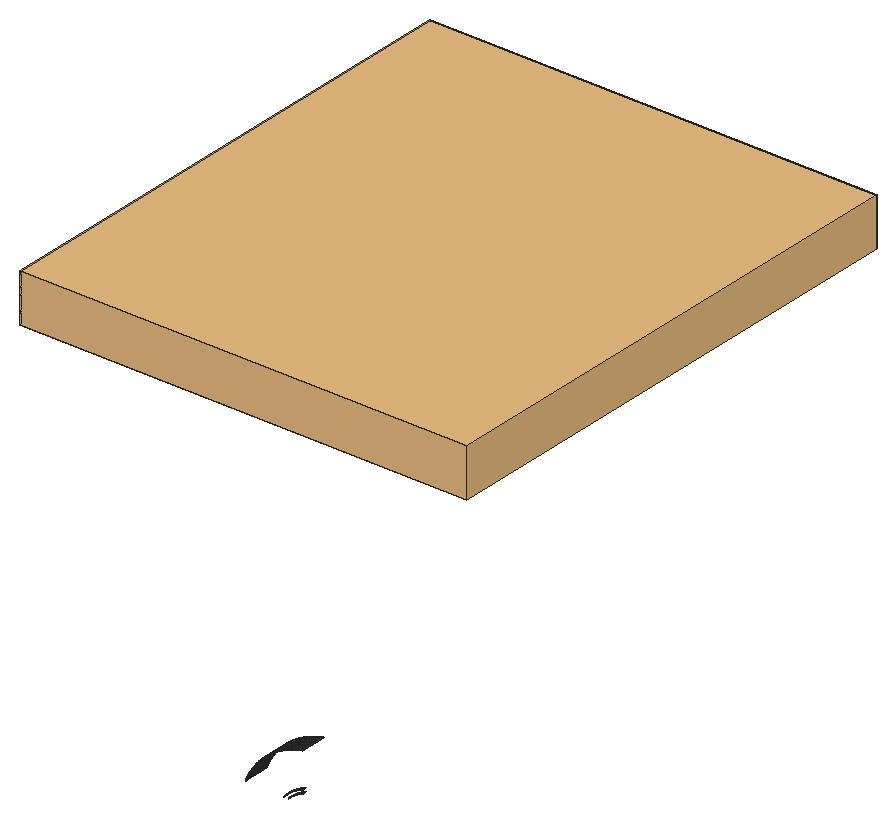
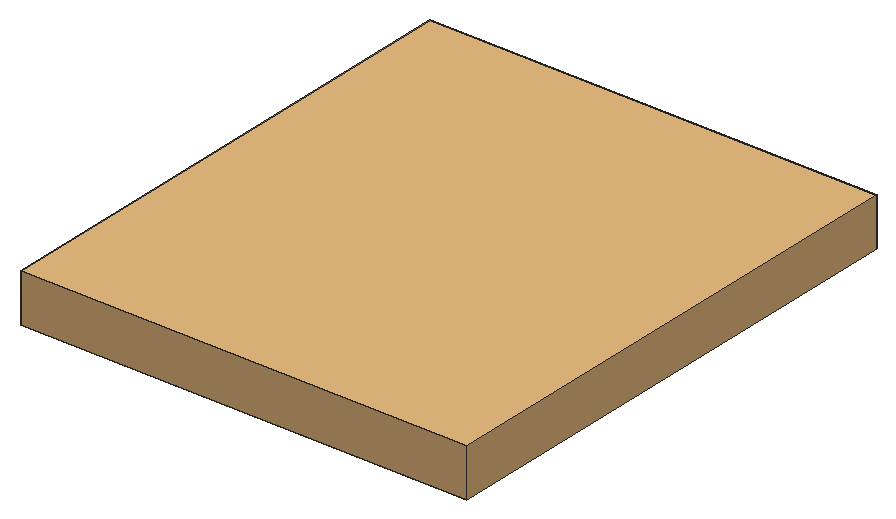
# SketchUp Ruby script. Lengths in inches.
U = 1.inch
M = Sketchup.active_model
def pt(a) = Geom::Point3d.new(a.map { |v| v * U })
def face(e, loops, mat)
  f = e.add_face(loops[0].map { |a| pt(a) })
  loops[1..].each { |l| e.add_face(l.map { |a| pt(a) }).erase! }
  f.material = f.back_material = mat if mat
  f
end
# faces: each face lists its corners as indices into pts; further lists are holes
def faces(e, pts, list, mat = nil) = list.each { |f| face(e, (f[0].is_a?(Array) ? f : [f]).map { |l| l.map { |i| pts[i] } }, mat) }
# xy, xz, yz: faces in a plane at the given z, y or x. An outline is a flat list of corners, or four numbers for a rectangle; further outlines are holes
def ring(l) = l.size == 4 ? [[l[0], l[1]], [l[2], l[1]], [l[2], l[3]], [l[0], l[3]]] : l.each_slice(2).to_a
def flat(e, list, mat, &to3) = list.each { |f| face(e, (f[0].is_a?(Array) ? f : [f]).map { |l| ring(l).map { |u, v| to3.(u, v) } }, mat) }
def xy(e, z, list, mat = nil) = flat(e, list, mat) { |x, y| [x, y, z] }
def xz(e, y, list, mat = nil) = flat(e, list, mat) { |x, z| [x, y, z] }
def yz(e, x, list, mat = nil) = flat(e, list, mat) { |y, z| [x, y, z] }
def lines(e, pts, list) = list.each { |a, b| e.add_line(pt(pts[a]), pt(pts[b])) }
# prism: a flat outline (further loops are holes) pulled along v
def prism(e, loops, v, mat = nil)
  f = face(e, loops, mat); d = Geom::Vector3d.new(v.map { |x| x * U })
  f.pushpull(f.normal.samedirection?(d) ? d.length : -d.length)
end
def box(e, o, s, mat = nil) = prism(e, [[o, [o[0] + s[0], o[1], o[2]], [o[0] + s[0], o[1] + s[1], o[2]], [o[0], o[1] + s[1], o[2]]]], [0, 0, s[2]], mat)
def at(x, y, z, deg = 0) = Geom::Transformation.translation(pt([x, y, z])) * Geom::Transformation.rotation(ORIGIN, Z_AXIS, deg.degrees)
def axes(o, x, y, z) = Geom::Transformation.new([*x, 0, *y, 0, *z, 0, *pt(o).to_a, 1])
def part(name) = M.definitions.add(name)
# library, detail: a bought-in or finely detailed component or shape, given as its bounding box
def library(name, o, s) = part(name).tap { |d| box(d.entities, o, s) }
def detail(e, o, s) = box(e.add_group.entities, o, s)
def put(e, d, t, mat = nil) = e.add_instance(d, t).tap { |i| i.material = mat if mat }
def group(e, t, mat = nil) = e.add_group.tap { |g| g.transformation = t; g.material = mat if mat }.entities
root = M.entities
M.materials.add("1432 AP 8245 TAR ROAD").color = [71, 72, 75]
M.materials.add("Outer Light").color = [251, 217, 152]
c1 = library("2",[-24,-36,-9.91],[204,234,21.91])
p = [[263.52,95.37,574.23],[263.41,95.37,574.11],[263.41,96.87,574.11],[263.52,96.87,574.23],[263.52,96.87,574.23],[263.41,96.87,574.11],
  [263.41,95.37,574.11],[263.52,95.37,574.23],[265.46,95.37,574.12],[265.56,95.37,574.23],[265.56,96.87,574.23],[265.46,96.87,574.12],
  [265.46,96.87,574.12],[265.56,96.87,574.23],[265.56,95.37,574.23],[265.46,95.37,574.12],[263.62,95.37,574.35],[263.62,96.87,574.35],
  [263.62,96.87,574.35],[263.62,95.37,574.35],[265.67,95.37,574.33],[265.67,96.87,574.33],[265.67,96.87,574.33],[265.67,95.37,574.33],
  [245.74,107.37,574.57],[245.63,107.37,574.31],[245.63,95.37,574.31],[245.74,95.37,574.57],[263.73,95.37,574.47],[263.73,96.87,574.47],
  [263.73,96.87,574.47],[263.73,95.37,574.47],[265.78,95.37,574.4375],[265.78,96.87,574.4375],[265.78,96.87,574.4375],[265.78,95.37,574.4375],
  [265.89,95.37,574.54],[265.89,96.87,574.54],[265.89,96.87,574.54],[265.89,95.37,574.54],[263.84,95.37,574.59],[263.84,96.87,574.59],
  [263.84,96.87,574.59],[263.84,95.37,574.59],[265.99,95.37,574.64],[265.99,96.87,574.64],[265.99,96.87,574.64],[265.99,95.37,574.64],
  [245.85,107.37,574.83],[245.85,95.37,574.83],[263.95,95.37,574.71],[263.95,96.87,574.71],[263.95,96.87,574.71],[263.95,95.37,574.71],
  [266.1,95.37,574.74],[266.1,96.87,574.74],[266.1,96.87,574.74],[266.1,95.37,574.74],[264.06,95.37,574.83],[264.06,96.87,574.83],
  [264.06,96.87,574.83],[264.06,95.37,574.83],[266.21,95.37,574.85],[266.21,96.87,574.85],[266.21,96.87,574.85],[266.21,95.37,574.85],
  [245.96,107.37,575.09],[245.96,95.37,575.09],[264.17,95.37,574.94],[264.17,96.87,574.94],[264.17,96.87,574.94],[264.17,95.37,574.94],
  [266.32,95.37,574.95],[266.32,96.87,574.95],[266.32,96.87,574.95],[266.32,95.37,574.95],[264.28,95.37,575.06],[264.28,96.87,575.06],
  [264.28,96.87,575.06],[264.28,95.37,575.06],[266.44,95.37,575.04],[266.44,96.87,575.04],[266.44,96.87,575.04],[266.44,95.37,575.04],
  [266.55,95.37,575.14],[266.55,96.87,575.14],[266.55,96.87,575.14],[266.55,95.37,575.14],[246.07,107.37,575.35],[246.07,95.37,575.35],
  [264.39,95.37,575.17],[264.39,96.87,575.17],[264.39,96.87,575.17],[264.39,95.37,575.17],[266.66,95.37,575.24],[266.66,96.87,575.24],
  [266.66,96.87,575.24],[266.66,95.37,575.24],[264.5,95.37,575.29],[264.5,96.87,575.29],[264.5,96.87,575.29],[264.5,95.37,575.29],
  [266.77,95.37,575.34],[266.77,96.87,575.34],[266.77,96.87,575.34],[266.77,95.37,575.34],[246.1875,107.37,575.61],[246.1875,95.37,575.61],
  [264.62,95.37,575.4],[264.62,96.87,575.4],[264.62,96.87,575.4],[264.62,95.37,575.4],[266.89,95.37,575.43],[266.89,96.87,575.43],
  [266.89,96.87,575.43],[266.89,95.37,575.43],[264.73,95.37,575.51],[264.73,96.87,575.51],[264.73,96.87,575.51],[264.73,95.37,575.51],
  [267,95.37,575.53],[267,96.87,575.53],[267,96.87,575.53],[267,95.37,575.53],[264.85,95.37,575.625],[264.85,96.87,575.625],
  [264.85,96.87,575.625],[264.85,95.37,575.625],[267.12,95.37,575.62],[267.12,96.87,575.62],[267.12,96.87,575.62],[267.12,95.37,575.62],
  [246.31,107.37,575.86],[246.31,95.37,575.86],[264.97,95.37,575.74],[264.97,96.87,575.74],[264.97,96.87,575.74],[264.97,95.37,575.74],
  [267.24,95.37,575.71],[267.24,96.87,575.71],[267.24,96.87,575.71],[267.24,95.37,575.71],[265.08,95.37,575.85],[265.08,96.87,575.85],
  [265.08,96.87,575.85],[265.08,95.37,575.85],[267.35,95.37,575.8],[267.35,96.87,575.8],[267.35,96.87,575.8],[267.35,95.37,575.8],
  [265.2,95.37,575.95],[265.2,96.87,575.95],[265.2,96.87,575.95],[265.2,95.37,575.95],[267.47,95.37,575.9],[267.47,96.87,575.9],
  [267.47,96.87,575.9],[267.47,95.37,575.9],[246.43,107.37,576.12],[246.43,95.37,576.12],[267.59,95.37,575.99],[267.59,96.87,575.99],
  [267.59,96.87,575.99],[267.59,95.37,575.99],[265.32,95.37,576.0625],[265.32,96.87,576.0625],[265.32,96.87,576.0625],[265.32,95.37,576.0625],
  [267.71,95.37,576.08],[267.71,96.87,576.08],[267.71,96.87,576.08],[267.71,95.37,576.08],[246.55,107.37,576.375],[246.55,95.37,576.375],
  [265.44,95.37,576.17],[265.44,96.87,576.17],[265.44,96.87,576.17],[265.44,95.37,576.17],[267.83,95.37,576.16],[267.83,96.87,576.16],
  [267.83,96.87,576.16],[267.83,95.37,576.16],[265.5625,95.37,576.28],[265.5625,96.87,576.28],[265.5625,96.87,576.28],[265.5625,95.37,576.28],
  [267.95,95.37,576.25],[267.95,96.87,576.25],[267.95,96.87,576.25],[267.95,95.37,576.25],[265.6875,95.37,576.38],[265.6875,96.87,576.38],
  [265.6875,96.87,576.38],[265.6875,95.37,576.38],[268.07,95.37,576.34],[268.07,96.87,576.34],[268.07,96.87,576.34],[268.07,95.37,576.34],
  [268.2,95.37,576.42],[268.2,96.87,576.42],[268.2,96.87,576.42],[268.2,95.37,576.42],[246.67,107.37,576.63],[246.67,95.37,576.63],
  [265.81,95.37,576.48],[265.81,96.87,576.48],[265.81,96.87,576.48],[265.81,95.37,576.48],[268.32,95.37,576.51],[268.32,96.87,576.51],
  [268.32,96.87,576.51],[268.32,95.37,576.51],[265.93,95.37,576.59],[265.93,96.87,576.59],[265.93,96.87,576.59],[265.93,95.37,576.59],
  [268.44,95.37,576.59],[268.44,96.87,576.59],[268.44,96.87,576.59],[268.44,95.37,576.59],[246.8,107.37,576.88],[246.8,95.37,576.88],
  [266.06,95.37,576.69],[266.06,96.87,576.69],[266.06,96.87,576.69],[266.06,95.37,576.69],[268.57,95.37,576.67],[268.57,96.87,576.67],
  [268.57,96.87,576.67],[268.57,95.37,576.67],[266.18,95.37,576.79],[266.18,96.87,576.79],[266.18,96.87,576.79],[266.18,95.37,576.79],
  [268.69,95.37,576.75],[268.69,96.87,576.75],[268.69,96.87,576.75],[268.69,95.37,576.75],[266.31,95.37,576.89],[266.31,96.87,576.89],
  [266.31,96.87,576.89],[266.31,95.37,576.89],[268.82,95.37,576.83],[268.82,96.87,576.83],[268.82,96.87,576.83],[268.82,95.37,576.83],
  [268.95,95.37,576.91],[268.95,96.87,576.91],[268.95,96.87,576.91],[268.95,95.37,576.91],[246.92,107.37,577.14],[246.92,95.37,577.14],
  [266.44,95.37,576.99],[266.44,96.87,576.99],[266.44,96.87,576.99],[266.44,95.37,576.99],[269.07,95.37,576.99],[269.07,96.87,576.99],
  [269.07,96.87,576.99],[269.07,95.37,576.99],[266.5625,95.37,577.09],[266.5625,96.87,577.09],[266.5625,96.87,577.09],[266.5625,95.37,577.09],
  [269.2,95.37,577.07],[269.2,96.87,577.07],[269.2,96.87,577.07],[269.2,95.37,577.07],[247.05,107.37,577.39],[247.05,95.37,577.39],
  [266.69,95.37,577.1875],[266.69,96.87,577.1875],[266.69,96.87,577.1875],[266.69,95.37,577.1875],[269.33,95.37,577.15],[269.33,96.87,577.15],
  [269.33,96.87,577.15],[269.33,95.37,577.15],[269.46,95.37,577.22],[269.46,96.87,577.22],[269.46,96.87,577.22],[269.46,95.37,577.22],
  [266.82,95.37,577.28],[266.82,96.87,577.28],[266.82,96.87,577.28],[266.82,95.37,577.28],[269.59,95.37,577.3],[269.59,96.87,577.3],
  [269.59,96.87,577.3],[269.59,95.37,577.3],[266.95,95.37,577.375],[266.95,96.87,577.375],[266.95,96.87,577.375],[266.95,95.37,577.375],
  [269.72,95.37,577.37],[269.72,96.87,577.37],[269.72,96.87,577.37],[269.72,95.37,577.37],[247.18,107.37,577.64],[247.18,95.37,577.64],
  [267.08,95.37,577.47],[267.08,96.87,577.47],[267.08,96.87,577.47],[267.08,95.37,577.47],[269.85,95.37,577.44],[269.85,96.87,577.44],
  [269.85,96.87,577.44],[269.85,95.37,577.44],[269.98,95.37,577.51],[269.98,96.87,577.51],[269.98,96.87,577.51],[269.98,95.37,577.51],
  [267.21,95.37,577.5625],[267.21,96.87,577.5625],[267.21,96.87,577.5625],[267.21,95.37,577.5625],[270.11,95.37,577.58],[270.11,96.87,577.58],
  [270.11,96.87,577.58],[270.11,95.37,577.58],[247.32,107.37,577.89],[247.32,95.37,577.89],[267.34,95.37,577.66],[267.34,96.87,577.66],
  [267.34,96.87,577.66],[267.34,95.37,577.66],[270.24,95.37,577.65],[270.24,96.87,577.65],[270.24,96.87,577.65],[270.24,95.37,577.65],
  [267.48,95.37,577.75],[267.48,96.87,577.75],[267.48,96.87,577.75],[267.48,95.37,577.75],[267.61,95.37,577.84],[267.61,96.87,577.84],
  [267.61,96.87,577.84],[267.61,95.37,577.84],[270.375,95.37,577.72],[270.375,96.87,577.72],[270.375,96.87,577.72],[270.375,95.37,577.72],
  [270.51,95.37,577.79],[270.51,96.87,577.79],[270.51,96.87,577.79],[270.51,95.37,577.79],[267.75,95.37,577.93],[267.75,96.87,577.93],
  [267.75,96.87,577.93],[267.75,95.37,577.93],[270.64,95.37,577.85],[270.64,96.87,577.85],[270.64,96.87,577.85],[270.64,95.37,577.85],
  [247.45,107.37,578.14],[247.45,95.37,578.14],[267.88,95.37,578.01],[267.88,96.87,578.01],[267.88,96.87,578.01],[267.88,95.37,578.01],
  [270.78,95.37,577.92],[270.78,96.87,577.92],[270.78,96.87,577.92],[270.78,95.37,577.92],[270.91,95.37,577.98],[270.91,96.87,577.98],
  [270.91,96.87,577.98],[270.91,95.37,577.98],[268.02,95.37,578.1],[268.02,96.87,578.1],[268.02,96.87,578.1],[268.02,95.37,578.1],
  [271.05,95.37,578.05],[271.05,96.87,578.05],[271.05,96.87,578.05],[271.05,95.37,578.05],[271.18,95.37,578.11],[271.18,96.87,578.11],
  [271.18,96.87,578.11],[271.18,95.37,578.11],[247.59,107.37,578.38],[247.59,95.37,578.38],[268.15,95.37,578.1875],[268.15,96.87,578.1875],
  [268.15,96.87,578.1875],[268.15,95.37,578.1875],[271.32,95.37,578.17],[271.32,96.87,578.17],[271.32,96.87,578.17],[271.32,95.37,578.17],
  [268.29,95.37,578.27],[268.29,96.87,578.27],[268.29,96.87,578.27],[268.29,95.37,578.27],[271.45,95.37,578.23],[271.45,96.87,578.23],
  [271.45,96.87,578.23],[271.45,95.37,578.23],[271.59,95.37,578.29],[271.59,96.87,578.29],[271.59,96.87,578.29],[271.59,95.37,578.29],
  [268.43,95.37,578.35],[268.43,96.87,578.35],[268.43,96.87,578.35],[268.43,95.37,578.35],[271.73,95.37,578.35],[271.73,96.87,578.35],
  [271.73,96.87,578.35],[271.73,95.37,578.35],[271.87,95.37,578.4],[271.87,96.87,578.4],[271.87,96.87,578.4],[271.87,95.37,578.4],
  [247.73,107.37,578.63],[247.73,95.37,578.63],[268.56,95.37,578.4375],[268.56,96.87,578.4375],[268.56,96.87,578.4375],[268.56,95.37,578.4375],
  [268.7,95.37,578.52],[268.7,96.87,578.52],[268.7,96.87,578.52],[268.7,95.37,578.52],[272.01,95.37,578.46],[272.01,96.87,578.46],
  [272.01,96.87,578.46],[272.01,95.37,578.46],[268.84,95.37,578.6],[268.84,96.87,578.6],[268.84,96.87,578.6],[268.84,95.37,578.6],
  [247.87,107.37,578.875],[247.87,95.37,578.875],[268.98,95.37,578.68],[268.98,96.87,578.68],[268.98,96.87,578.68],[268.98,95.37,578.68],
  [269.125,95.37,578.76],[269.125,96.87,578.76],[269.125,96.87,578.76],[269.125,95.37,578.76],[269.27,95.37,578.83],[269.27,96.87,578.83],
  [269.27,96.87,578.83],[269.27,95.37,578.83],[269.41,95.37,578.91],[269.41,96.87,578.91],[269.41,96.87,578.91],[269.41,95.37,578.91],
  [248.01,107.37,579.12],[248.01,95.37,579.12],[269.55,95.37,578.98],[269.55,96.87,578.98],[269.55,96.87,578.98],[269.55,95.37,578.98],
  [269.69,95.37,579.06],[269.69,96.87,579.06],[269.69,96.87,579.06],[269.69,95.37,579.06],[248.16,107.37,579.36],[248.16,95.37,579.36],
  [269.84,95.37,579.13],[269.84,96.87,579.13],[269.84,96.87,579.13],[269.84,95.37,579.13],[269.98,95.37,579.2],[269.98,96.87,579.2],
  [269.98,96.87,579.2],[269.98,95.37,579.2],[270.125,95.37,579.27],[270.125,96.87,579.27],[270.125,96.87,579.27],[270.125,95.37,579.27],
  [270.27,95.37,579.34],[270.27,96.87,579.34],[270.27,96.87,579.34],[270.27,95.37,579.34],[270.42,95.37,579.41],[270.42,96.87,579.41],
  [270.42,96.87,579.41],[270.42,95.37,579.41],[248.3,107.37,579.6],[248.3,95.37,579.6],[270.5625,95.37,579.48],[270.5625,96.87,579.48],
  [270.5625,96.87,579.48],[270.5625,95.37,579.48],[270.71,95.37,579.54],[270.71,96.87,579.54],[270.71,96.87,579.54],[270.71,95.37,579.54],
  [270.86,95.37,579.61],[270.86,96.87,579.61],[270.86,96.87,579.61],[270.86,95.37,579.61],[248.45,107.37,579.84],[248.45,95.37,579.84],
  [271.01,95.37,579.67],[271.01,96.87,579.67],[271.01,96.87,579.67],[271.01,95.37,579.67],[271.15,95.37,579.73],[271.15,96.87,579.73],
  [271.15,96.87,579.73],[271.15,95.37,579.73],[271.3,95.37,579.79],[271.3,96.87,579.79],[271.3,96.87,579.79],[271.3,95.37,579.79],
  [248.6,107.37,580.08],[248.6,95.37,580.08],[271.45,95.37,579.85],[271.45,96.87,579.85],[271.45,96.87,579.85],[271.45,95.37,579.85],
  [271.6,95.37,579.91],[271.6,96.87,579.91],[271.6,96.87,579.91],[271.6,95.37,579.91],[271.75,95.37,579.97],[271.75,96.87,579.97],
  [271.75,96.87,579.97],[271.75,95.37,579.97],[271.9,95.37,580.02],[271.9,96.87,580.02],[271.9,96.87,580.02],[271.9,95.37,580.02],
  [272.06,95.37,580.08],[272.06,96.87,580.08],[248.76,107.37,580.32],[248.76,95.37,580.32],[248.91,107.37,580.56],[248.91,95.37,580.56],
  [249.07,107.37,580.79],[249.07,95.37,580.79],[249.23,107.37,581.03],[249.23,95.37,581.03],[249.38,107.37,581.26],[249.38,95.37,581.26],
  [249.55,107.37,581.49],[249.55,95.37,581.49],[249.71,107.37,581.72],[249.71,95.37,581.72],[249.875,107.37,581.95],[249.875,95.37,581.95],
  [250.04,107.37,582.18],[250.04,95.37,582.18],[250.21,107.37,582.41],[250.21,95.37,582.41],[250.38,107.37,582.63],[250.38,95.37,582.63],
  [250.55,107.37,582.86],[250.55,95.37,582.86],[250.73,107.37,583.08],[250.73,95.37,583.08],[250.9,107.37,583.3],[250.9,95.37,583.3],
  [251.08,107.37,583.52],[251.08,95.37,583.52],[251.26,107.37,583.74],[251.26,95.37,583.74],[251.44,107.37,583.96],[251.44,95.37,583.96],
  [251.625,107.37,584.17],[251.625,95.37,584.17],[251.81,107.37,584.39],[251.81,95.37,584.39],[252,107.37,584.6],[252,95.37,584.6],
  [252.18,107.37,584.8125],[252.18,95.37,584.8125],[252.375,107.37,585.02],[252.375,95.37,585.02],[252.5625,107.37,585.23],[252.5625,95.37,585.23],
  [252.76,107.37,585.4375],[252.76,95.37,585.4375],[252.95,107.37,585.64],[252.95,95.37,585.64],[253.15,107.37,585.84],[253.15,95.37,585.84],
  [253.35,107.37,586.05],[253.35,95.37,586.05],[253.54,107.37,586.25],[253.54,95.37,586.25],[253.74,107.37,586.45],[253.74,95.37,586.45],
  [253.95,107.37,586.64],[253.95,95.37,586.64],[254.15,107.37,586.84],[254.15,95.37,586.84],[254.36,107.37,587.03],[254.36,95.37,587.03],
  [254.5625,107.37,587.23],[254.5625,95.37,587.23],[254.77,107.37,587.42],[254.77,95.37,587.42],[254.98,107.37,587.61],[254.98,95.37,587.61],
  [255.19,107.37,587.8],[255.19,95.37,587.8],[255.41,107.37,587.98],[255.41,95.37,587.98],[255.62,107.37,588.17],[255.62,95.37,588.17],
  [255.84,107.37,588.35],[255.84,95.37,588.35],[256.05,107.37,588.53],[256.05,95.37,588.53],[256.27,107.37,588.71],[256.27,95.37,588.71],
  [256.49,107.37,588.89],[256.49,95.37,588.89],[256.71,107.37,589.0625],[256.71,95.37,589.0625],[256.94,107.37,589.24],[256.94,95.37,589.24],
  [257.16,107.37,589.41],[257.16,95.37,589.41],[257.38,107.37,589.58],[257.38,95.37,589.58],[257.61,107.37,589.75],[257.61,95.37,589.75],
  [257.84,107.37,589.92],[257.84,95.37,589.92],[258.07,107.37,590.08],[258.07,95.37,590.08],[258.3,107.37,590.25],[258.3,95.37,590.25],
  [258.53,107.37,590.41],[258.53,95.37,590.41],[258.76,107.37,590.57],[258.76,95.37,590.57],[259,107.37,590.72],[259,95.37,590.72],
  [259.24,107.37,590.88],[259.24,95.37,590.88],[259.47,107.37,591.04],[259.47,95.37,591.04],[259.71,107.37,591.1875],[259.71,95.37,591.1875],
  [259.95,107.37,591.34],[259.95,95.37,591.34],[260.19,107.37,591.49],[260.19,95.37,591.49],[260.43,107.37,591.63],[260.43,95.37,591.63],
  [260.67,107.37,591.78],[260.67,95.37,591.78],[260.92,107.37,591.92],[260.92,95.37,591.92],[261.16,107.37,592.0625],[261.16,95.37,592.0625],
  [261.41,107.37,592.2],[261.41,95.37,592.2],[261.66,107.37,592.34],[261.66,95.37,592.34],[261.91,107.37,592.47],[261.91,95.37,592.47],
  [262.15,107.37,592.61],[262.15,95.37,592.61],[262.4,107.37,592.74],[262.4,95.37,592.74],[262.66,107.37,592.87],[262.66,95.37,592.87],
  [262.91,107.37,593],[262.91,95.37,593],[263.16,107.37,593.12],[263.16,95.37,593.12],[263.42,107.37,593.24],[263.42,95.37,593.24],
  [263.67,107.37,593.37],[263.67,95.37,593.37],[263.93,107.37,593.49],[263.93,95.37,593.49],[264.19,107.37,593.6],[264.19,95.37,593.6],
  [264.44,107.37,593.72],[264.44,95.37,593.72],[264.7,107.37,593.83],[264.7,95.37,593.83],[264.96,107.37,593.94],[264.96,95.37,593.94],
  [265.22,107.37,594.05],[265.22,95.37,594.05],[265.49,107.37,594.16],[265.49,95.37,594.16],[265.75,107.37,594.26],[265.75,95.37,594.26],
  [266.01,107.37,594.37],[266.01,95.37,594.37],[266.27,107.37,594.47],[266.27,95.37,594.47],[266.54,107.37,594.57],[266.54,95.37,594.57],
  [266.81,107.37,594.66],[266.81,95.37,594.66],[267.07,107.37,594.76],[267.07,95.37,594.76],[267.34,107.37,594.85],[267.34,95.37,594.85],
  [267.61,107.37,594.94],[267.61,95.37,594.94],[267.875,107.37,595.03],[267.875,95.37,595.03],[268.14,107.37,595.12],[268.14,95.37,595.12],
  [268.41,107.37,595.2],[268.41,95.37,595.2],[268.69,107.37,595.28],[268.69,95.37,595.28],[268.96,107.37,595.36],[268.96,95.37,595.36],
  [269.23,107.37,595.44],[269.23,95.37,595.44],[269.5,107.37,595.52],[269.5,95.37,595.52],[269.77,107.37,595.59],[269.77,95.37,595.59],
  [270.05,107.37,595.66],[270.05,95.37,595.66],[270.32,107.37,595.73],[270.32,95.37,595.73],[270.6,107.37,595.8],[270.6,95.37,595.8],
  [270.87,107.37,595.86],[270.87,95.37,595.86],[271.15,107.37,595.93],[271.15,95.37,595.93],[271.42,107.37,595.99],[271.42,95.37,595.99],
  [271.7,107.37,596.04],[271.7,95.37,596.04],[271.98,107.37,596.1],[271.98,95.37,596.1]]
faces(root,p,[[0,1,2,3],[8,9,10,11],[16,0,3,17],[9,20,21,10],[24,25,26,27],[28,16,17,29],[20,32,33,21],[32,36,37,33],
  [40,28,29,41],[36,44,45,37],[48,24,27,49],[50,40,41,51],[44,54,55,45],[58,50,51,59],[54,62,63,55],[66,48,49,67],
  [68,58,59,69],[62,72,73,63],[76,68,69,77],[72,80,81,73],[80,84,85,81],[88,66,67,89],[90,76,77,91],[84,94,95,85],
  [98,90,91,99],[94,102,103,95],[106,88,89,107],[108,98,99,109],[102,112,113,103],[116,108,109,117],[112,120,121,113],[124,116,117,125],
  [120,128,129,121],[132,106,107,133],[134,124,125,135],[128,138,139,129],[142,134,135,143],[138,146,147,139],[150,142,143,151],[146,154,155,147],
  [158,132,133,159],[154,160,161,155],[164,150,151,165],[160,168,169,161],[172,158,159,173],[174,164,165,175],[168,178,179,169],[182,174,175,183],
  [178,186,187,179],[190,182,183,191],[186,194,195,187],[194,198,199,195],[202,172,173,203],[204,190,191,205],[198,208,209,199],[212,204,205,213],
  [208,216,217,209],[220,202,203,221],[222,212,213,223],[216,226,227,217],[230,222,223,231],[226,234,235,227],[238,230,231,239],[234,242,243,235],
  [242,246,247,243],[250,220,221,251],[252,238,239,253],[246,256,257,247],[260,252,253,261],[256,264,265,257],[268,250,251,269],[270,260,261,271],
  [264,274,275,265],[274,278,279,275],[282,270,271,283],[278,286,287,279],[290,282,283,291],[286,294,295,287],[298,268,269,299],[300,290,291,301],
  [294,304,305,295],[304,308,309,305],[312,300,301,313],[308,316,317,309],[320,298,299,321],[322,312,313,323],[316,326,327,317],[330,322,323,331],
  [334,330,331,335],[326,338,339,327],[338,342,343,339],[346,334,335,347],[342,350,351,343],[354,320,321,355],[356,346,347,357],[350,360,361,351],
  [360,364,365,361],[368,356,357,369],[364,372,373,365],[372,376,377,373],[380,354,355,381],[382,368,369,383],[376,386,387,377],[390,382,383,391],
  [386,394,395,387],[394,398,399,395],[402,390,391,403],[398,406,407,399],[406,410,411,407],[414,380,381,415],[416,402,403,417],[420,416,417,421],
  [410,424,425,411],[428,420,421,429],[432,414,415,433],[434,428,429,435],[438,434,435,439],[442,438,439,443],[446,442,443,447],[450,432,433,451],
  [452,446,447,453],[456,452,453,457],[460,450,451,461],[462,456,457,463],[466,462,463,467],[470,466,467,471],[474,470,471,475],[478,474,475,479],
  [482,460,461,483],[484,478,479,485],[488,484,485,489],[492,488,489,493],[496,482,483,497],[498,492,493,499],[502,498,499,503],[506,502,503,507],
  [510,496,497,511],[512,506,507,513],[516,512,513,517],[520,516,517,521],[524,520,521,525],[528,524,525,529],[530,510,511,531],[532,530,531,533],
  [534,532,533,535],[536,534,535,537],[538,536,537,539],[540,538,539,541],[542,540,541,543],[544,542,543,545],[546,544,545,547],[548,546,547,549],
  [550,548,549,551],[552,550,551,553],[554,552,553,555],[556,554,555,557],[558,556,557,559],[560,558,559,561],[562,560,561,563],[564,562,563,565],
  [566,564,565,567],[568,566,567,569],[570,568,569,571],[572,570,571,573],[574,572,573,575],[576,574,575,577],[578,576,577,579],[580,578,579,581],
  [582,580,581,583],[584,582,583,585],[586,584,585,587],[588,586,587,589],[590,588,589,591],[592,590,591,593],[594,592,593,595],[596,594,595,597],
  [598,596,597,599],[600,598,599,601],[602,600,601,603],[604,602,603,605],[606,604,605,607],[608,606,607,609],[610,608,609,611],[612,610,611,613],
  [614,612,613,615],[616,614,615,617],[618,616,617,619],[620,618,619,621],[622,620,621,623],[624,622,623,625],[626,624,625,627],[628,626,627,629],
  [630,628,629,631],[632,630,631,633],[634,632,633,635],[636,634,635,637],[638,636,637,639],[640,638,639,641],[642,640,641,643],[644,642,643,645],
  [646,644,645,647],[648,646,647,649],[650,648,649,651],[652,650,651,653],[654,652,653,655],[656,654,655,657],[658,656,657,659],[660,658,659,661],
  [662,660,661,663],[664,662,663,665],[666,664,665,667],[668,666,667,669],[670,668,669,671],[672,670,671,673],[674,672,673,675],[676,674,675,677],
  [678,676,677,679],[680,678,679,681],[682,680,681,683],[684,682,683,685],[686,684,685,687],[688,686,687,689],[690,688,689,691],[692,690,691,693],
  [694,692,693,695],[696,694,695,697],[698,696,697,699],[700,698,699,701],[702,700,701,703],[704,702,703,705],[706,704,705,707],[708,706,707,709],
  [710,708,709,711],[712,710,711,713],[714,712,713,715],[716,714,715,717],[718,716,717,719],[720,718,719,721],[722,720,721,723],[724,722,723,725],
  [726,724,725,727],[728,726,727,729],[730,728,729,731],[732,730,731,733],[734,732,733,735]],"1432 AP 8245 TAR ROAD")
faces(root,p,[[4,5,6,7],[12,13,14,15],[18,4,7,19],[13,22,23,14],[30,18,19,31],[22,34,35,23],[34,38,39,35],[42,30,31,43],
  [38,46,47,39],[52,42,43,53],[46,56,57,47],[60,52,53,61],[56,64,65,57],[70,60,61,71],[64,74,75,65],[78,70,71,79],
  [74,82,83,75],[82,86,87,83],[92,78,79,93],[86,96,97,87],[100,92,93,101],[96,104,105,97],[110,100,101,111],[104,114,115,105],
  [118,110,111,119],[114,122,123,115],[126,118,119,127],[122,130,131,123],[136,126,127,137],[130,140,141,131],[144,136,137,145],[140,148,149,141],
  [152,144,145,153],[148,156,157,149],[156,162,163,157],[166,152,153,167],[162,170,171,163],[176,166,167,177],[170,180,181,171],[184,176,177,185],
  [180,188,189,181],[192,184,185,193],[188,196,197,189],[196,200,201,197],[206,192,193,207],[200,210,211,201],[214,206,207,215],[210,218,219,211],
  [224,214,215,225],[218,228,229,219],[232,224,225,233],[228,236,237,229],[240,232,233,241],[236,244,245,237],[244,248,249,245],[254,240,241,255],
  [248,258,259,249],[262,254,255,263],[258,266,267,259],[272,262,263,273],[266,276,277,267],[276,280,281,277],[284,272,273,285],[280,288,289,281],
  [292,284,285,293],[288,296,297,289],[302,292,293,303],[296,306,307,297],[306,310,311,307],[314,302,303,315],[310,318,319,311],[324,314,315,325],
  [318,328,329,319],[332,324,325,333],[336,332,333,337],[328,340,341,329],[340,344,345,341],[348,336,337,349],[344,352,353,345],[358,348,349,359],
  [352,362,363,353],[362,366,367,363],[370,358,359,371],[366,374,375,367],[374,378,379,375],[384,370,371,385],[378,388,389,379],[392,384,385,393],
  [388,396,397,389],[396,400,401,397],[404,392,393,405],[400,408,409,401],[408,412,413,409],[418,404,405,419],[422,418,419,423],[412,426,427,413],
  [430,422,423,431],[436,430,431,437],[440,436,437,441],[444,440,441,445],[448,444,445,449],[454,448,449,455],[458,454,455,459],[464,458,459,465],
  [468,464,465,469],[472,468,469,473],[476,472,473,477],[480,476,477,481],[486,480,481,487],[490,486,487,491],[494,490,491,495],[500,494,495,501],
  [504,500,501,505],[508,504,505,509],[514,508,509,515],[518,514,515,519],[522,518,519,523],[526,522,523,527]],"Outer Light")
put(root,c1,at(90,227.37,665.79))
